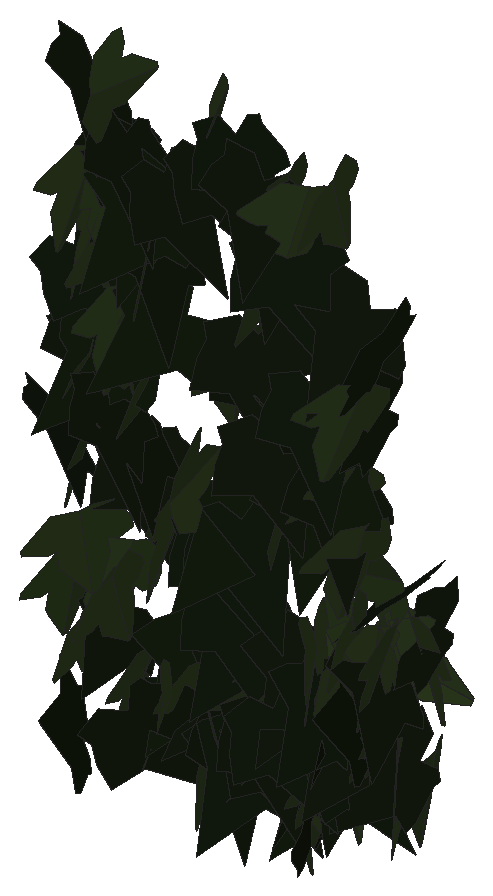
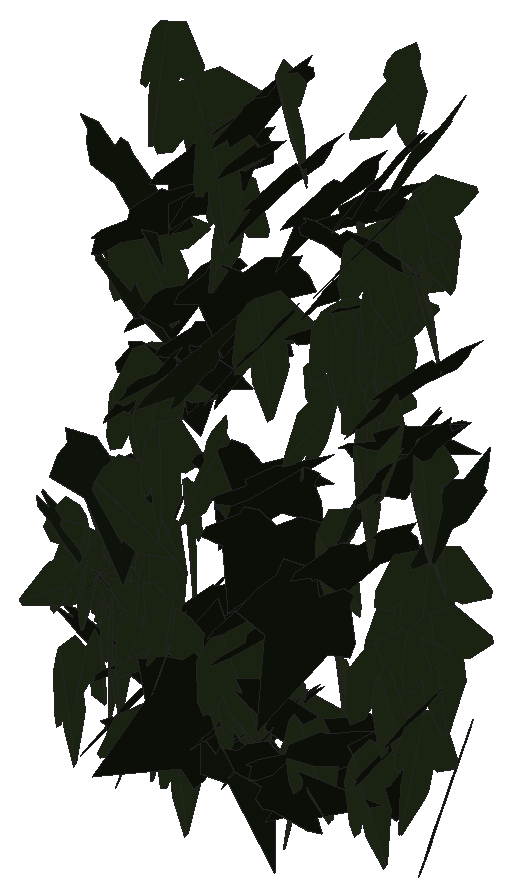
# SketchUp Ruby script. Lengths in inches.
U = 1.inch
M = Sketchup.active_model
def pt(a) = Geom::Point3d.new(a.map { |v| v * U })
def face(e, loops, mat)
  f = e.add_face(loops[0].map { |a| pt(a) })
  loops[1..].each { |l| e.add_face(l.map { |a| pt(a) }).erase! }
  f.material = f.back_material = mat if mat
  f
end
# faces: each face lists its corners as indices into pts; further lists are holes
def faces(e, pts, list, mat = nil) = list.each { |f| face(e, (f[0].is_a?(Array) ? f : [f]).map { |l| l.map { |i| pts[i] } }, mat) }
# xy, xz, yz: faces in a plane at the given z, y or x. An outline is a flat list of corners, or four numbers for a rectangle; further outlines are holes
def ring(l) = l.size == 4 ? [[l[0], l[1]], [l[2], l[1]], [l[2], l[3]], [l[0], l[3]]] : l.each_slice(2).to_a
def flat(e, list, mat, &to3) = list.each { |f| face(e, (f[0].is_a?(Array) ? f : [f]).map { |l| ring(l).map { |u, v| to3.(u, v) } }, mat) }
def xy(e, z, list, mat = nil) = flat(e, list, mat) { |x, y| [x, y, z] }
def xz(e, y, list, mat = nil) = flat(e, list, mat) { |x, z| [x, y, z] }
def yz(e, x, list, mat = nil) = flat(e, list, mat) { |y, z| [x, y, z] }
def lines(e, pts, list) = list.each { |a, b| e.add_line(pt(pts[a]), pt(pts[b])) }
# prism: a flat outline (further loops are holes) pulled along v
def prism(e, loops, v, mat = nil)
  f = face(e, loops, mat); d = Geom::Vector3d.new(v.map { |x| x * U })
  f.pushpull(f.normal.samedirection?(d) ? d.length : -d.length)
end
def box(e, o, s, mat = nil) = prism(e, [[o, [o[0] + s[0], o[1], o[2]], [o[0] + s[0], o[1] + s[1], o[2]], [o[0], o[1] + s[1], o[2]]]], [0, 0, s[2]], mat)
def at(x, y, z, deg = 0) = Geom::Transformation.translation(pt([x, y, z])) * Geom::Transformation.rotation(ORIGIN, Z_AXIS, deg.degrees)
def axes(o, x, y, z) = Geom::Transformation.new([*x, 0, *y, 0, *z, 0, *pt(o).to_a, 1])
def part(name) = M.definitions.add(name)
# library, detail: a bought-in or finely detailed component or shape, given as its bounding box
def library(name, o, s) = part(name).tap { |d| box(d.entities, o, s) }
def detail(e, o, s) = box(e.add_group.entities, o, s)
def put(e, d, t, mat = nil) = e.add_instance(d, t).tap { |i| i.material = mat if mat }
def group(e, t, mat = nil) = e.add_group.tap { |g| g.transformation = t; g.material = mat if mat }.entities
root = M.entities
M.materials.add("efeu1").color = [18, 25, 13]
M.materials.add("efeu2").color = [43, 57, 29]
c1 = part("ivyleaf_10")
p = [[0,0.5,-0.03],[-0.0625,2.02,-0.43],[-0.19,2.01,-0.46],[-0.54,1.05,-0.29],[-0.52,0.625,-0.18],[-0.83,0.76,-0.28],
  [-1.16,0.64,-0.33],[-1.15,0.33,-0.24],[-0.77,-0.39,0.02],[-0.3,-0.51,0.16],[0.04,-0.48,0.23],[-0.02,2.01,-0.4375],
  [-0.06,2.01,-0.43],[0.04,-0.49,0.23],[0.67,-0.49,0.14],[1.38,0.36,-0.2],[1.375,0.51,-0.24],[0.81,0.65,-0.19],
  [0.62,0.59,-0.15],[0.6,1.09,-0.28],[0.5,1.23,-0.31]]
faces(c1.entities,p,[[0,1,2,3,4,5,6,7,8,9,10],[11,12,0,13,14,15,16,17,18,19,20]],"efeu2")
c2 = part("ivyleaf_9")
p = [[1.54,2.16,1.25],[1.36,2.04,1.19],[-0.21,0.99,0.68],[-0.71,1.11,0.82],[-0.85,0.86,0.67],[-0.8,0.17,0.21],
  [-0.9,-0.01,0.1],[-0.67,-0.16,-0.02],[-0.08,-0.08,-0.05],[-0.03,-0.6,-0.4],[0.65,-0.88,-0.66],[0.83,-0.6,-0.49],
  [1.29,-0.42,-0.43],[1.8125,-0.07,-0.26],[1.21,0.44,0.15]]
faces(c2.entities,p,[[0,1,2,3,4,5,6,7,8,9,10,11,12,13,14]],"efeu1")
put(root,c1,axes([27.02,222.2,235.84],[0.27164,-0.32229,-0.26896],[-0.09984,0.26157,-0.41426],[0.40773,0.27877,0.07775]))
put(root,c2,axes([24.59,222.71,240.35],[-0.29862,-0.35269,0.19088],[-0.03799,-0.21204,-0.45121],[0.39923,-0.28399,0.09984]))
put(root,c1,axes([23.69,222.52,240.5625],[-0.01097,-0.47184,0.16507],[0.03742,-0.16543,-0.47036],[0.49848,0.00203,0.03894]))
put(root,c1,axes([24.21,222.51,239.03],[-0.03517,-0.47829,0.14144],[0.08713,-0.1455,-0.47036],[0.49109,-0.00844,0.09358]))
put(root,c2,axes([26.46,222.32,234.88],[0.08252,-0.39457,-0.29582],[-0.00101,0.29979,-0.40015],[0.49314,0.06664,0.04868]))
put(root,c1,axes([27.39,222.5,238.9375],[-0.15374,-0.44872,0.15817],[-0.03284,-0.15581,-0.47397],[0.47464,-0.15613,0.01844]))
put(root,c2,axes([26.36,222.43,238.18],[-0.08203,-0.40902,-0.27564],[0.09548,0.26097,-0.41566],[0.4839,-0.12083,0.03529]))
put(root,c2,axes([24.82,222.77,238.98],[-0.32782,-0.29622,0.23407],[-0.06945,-0.25739,-0.423],[0.37109,-0.30985,0.12761]))
put(root,c2,axes([25.96,222.71,241.03],[-0.03709,-0.47389,0.15508],[0.02325,-0.15698,-0.47415],[0.49808,-0.02796,0.03368]))
put(root,c1,axes([23.78,222.35,236.26],[-0.27606,-0.40929,-0.07917],[0.04487,0.06523,-0.49369],[0.41446,-0.27969,0.00071]))
put(root,c1,axes([24.96,222.26,234.52],[0.17602,-0.36599,-0.29167],[-0.13615,0.25809,-0.40602],[0.44775,0.22236,-0.0088]))
put(root,c1,axes([25.43,222.04,237.35],[0.02628,-0.01844,0.49897],[-0.24153,0.43684,0.02886],[-0.437,-0.24255,0.01406]))
put(root,c2,axes([27.27,222.76,234.82],[-0.08751,-0.04047,0.49062],[-0.0735,-0.49165,-0.05367],[0.48676,-0.08152,0.0801]))
put(root,c2,axes([23.18,222.71,237.16],[0.10075,-0.36999,0.32087],[0.15594,-0.28631,-0.3791],[0.46426,0.17646,0.0577]))
put(root,c2,axes([23.42,222.76,233.37],[-0.09246,-0.01791,0.49105],[-0.04589,-0.49717,-0.02677],[0.48923,-0.05002,0.0903]))
put(root,c2,axes([25.73,222.82,236.79],[-0.29562,-0.3588,0.18405],[-0.02742,-0.20979,-0.45303],[0.40231,-0.27794,0.10436]))
put(root,c2,axes([26.95,222.63,237.78],[-0.36102,-0.29576,-0.17942],[0.14103,0.11095,-0.46669],[0.31587,-0.38758,0.00331]))
put(root,c2,axes([23.9375,222.63,237.71],[0.15387,-0.47573,-0.00212],[-0.00062,0.00203,-0.5],[0.47574,0.15387,0.00003]))
put(root,c2,axes([26.78,222.54,233.38],[-0.01465,0.3683,0.33784],[-0.12204,-0.33039,0.35489],[0.48466,-0.07206,0.09958]))
put(root,c2,axes([26.75,222.65,238.7],[0.00917,-0.49319,-0.08172],[0.00753,0.08186,-0.4932],[0.49986,0.00781,0.00893]))
put(root,c1,axes([24.56,222.41,239.8125],[0.28014,-0.36912,-0.18781],[-0.06124,0.18733,-0.45952],[0.4096,0.28046,0.05975]))
put(root,c2,axes([27.91,222.3,239.73],[-0.23527,0.41139,0.15939],[-0.09462,0.12938,-0.47361],[-0.43092,-0.25301,0.01697]))
put(root,c2,axes([25.73,222.875,233.9],[-0.17539,-0.41991,0.20715],[-0.02601,-0.21213,-0.45202],[0.46751,-0.16933,0.05257]))
put(root,c1,axes([23.52,222.55,235.63],[-0.07759,-0.49393,-0.00373],[0.00149,0.00354,-0.49999],[0.49394,-0.0776,0.00092]))
put(root,c1,axes([27.36,222.6,237.19],[-0.09582,-0.48732,0.05775],[-0.01051,-0.05679,-0.49665],[0.49062,-0.0964,0.00064]))
put(root,c2,axes([26.71,222.93,234.78],[-0.12651,-0.36116,0.32181],[-0.01217,-0.33015,-0.3753],[0.48358,-0.1028,0.07474]))
put(root,c1,axes([24.2,222.43,239.84],[-0.18172,-0.43005,-0.17899],[0.05797,0.16976,-0.46671],[0.46219,-0.19037,-0.01184]))
put(root,c1,axes([26.44,222.81,233.54],[0.06044,-0.08595,-0.48883],[0.28794,-0.39504,0.10506],[-0.40428,-0.29421,0.00175]))
put(root,c2,axes([25.8,222.5625,236.86],[-0.20522,-0.25885,-0.37534],[0.24055,0.28819,-0.33027],[0.38732,-0.31614,0.00625]))
put(root,c2,axes([24.1,222.72,240.95],[0.13924,-0.48001,0.0141],[0.00413,-0.01348,-0.4998],[0.4802,0.1393,0.00021]))
put(root,c1,axes([24.16,222.19,241.82],[-0.00716,-0.11697,-0.48607],[0.08913,0.47804,-0.11635],[0.49194,-0.08831,0.014]))
put(root,c1,axes([24.12,222.45,235.57],[-0.02081,-0.45202,-0.21272],[0.03296,0.2112,-0.45201],[0.49848,-0.03284,0.02101]))
put(root,c1,axes([27.62,222.74,235.97],[0.21044,-0.43276,0.13578],[0.04232,-0.13029,-0.48087],[0.45158,0.21388,-0.01821]))
put(root,c2,axes([25.9375,222.68,239.12],[-0.12272,-0.42627,-0.23073],[0.06796,0.22053,-0.44356],[0.47992,-0.14023,0.00381]))
put(root,c1,axes([23.66,222.64,239.83],[0.31119,-0.39056,-0.02505],[-0.01242,0.02213,-0.49936],[0.39116,0.31141,0.00407]))
put(root,c2,axes([26.33,222.61,240.42],[0.0229,-0.42507,-0.26229],[0.01937,0.26312,-0.42473],[0.4991,0.00929,0.02851]))
put(root,c2,axes([24.4375,222.83,239.78],[0.07969,-0.48968,0.06217],[0.01451,-0.06062,-0.4961],[0.4934,0.08087,0.00455]))
put(root,c1,axes([26.52,222.71,240.99],[-0.26444,-0.4039,0.13012],[-0.03098,-0.13453,-0.48056],[0.42321,-0.26223,0.04612]))
put(root,c2,axes([26.95,222.83,237.68],[0.01658,-0.49941,-0.01778],[-0.00304,0.01769,-0.49968],[0.49972,0.01668,-0.00245]))
put(root,c1,axes([23.56,222.72,237.24],[0.25419,-0.42943,0.03129],[0.00758,-0.03187,-0.49893],[0.4305,0.25412,-0.00969]))
put(root,c2,axes([25.4375,222.9,233.99],[0.0901,-0.48493,0.08199],[0.00838,-0.08183,-0.49319],[0.49174,0.09025,-0.00662]))
put(root,c1,axes([27.04,222.56,241.38],[0.0352,-0.45479,-0.20476],[0.03648,0.20706,-0.45365],[0.49742,0.01699,0.04776]))
put(root,c2,axes([23.42,222.98,241.47],[0.07823,-0.44138,0.22151],[0.06292,-0.21354,-0.44771],[0.48982,0.09793,0.02213]))
put(root,c2,axes([25.98,222.78,234.43],[0.08024,-0.4752,-0.13322],[0.01057,0.13659,-0.48087],[0.49341,0.07435,0.03197]))
put(root,c2,axes([27.36,223.01,235.4375],[0.01548,-0.45973,0.19597],[0.03998,-0.1943,-0.45897],[0.49816,0.02988,0.03075]))
put(root,c2,axes([25.55,222.79,241.4],[0.11965,-0.47132,-0.11638],[-0.03302,0.11168,-0.48625],[0.48435,0.12404,-0.00441]))
put(root,c1,axes([24.27,222.81,239.03],[-0.07032,-0.48677,0.09007],[-0.01075,-0.08945,-0.49182],[0.49491,-0.0711,0.00211]))
put(root,c1,axes([24.61,222.92,236.46],[0.16594,-0.41447,0.22512],[0.0942,-0.20471,-0.44634],[0.46216,0.19054,0.01014]))
put(root,c2,axes([24.34,222.51,234.05],[-0.00426,-0.10556,-0.48871],[0.1696,0.45945,-0.10072],[0.47034,-0.16663,0.0319]))
put(root,c2,axes([26.4,223.09,235.16],[-0.19912,-0.42217,0.17922],[-0.03138,-0.18239,-0.46449],[0.45757,-0.19622,0.04614]))
put(root,c1,axes([26.16,222.55,239.93],[-0.00152,-0.40118,-0.29841],[0.00883,0.29835,-0.40114],[0.49992,-0.00648,0.00618]))
put(root,c1,axes([26.68,222.84,234.08],[0.12287,-0.4803,0.06492],[0.01082,-0.06424,-0.49574],[0.48455,0.12323,-0.00539]))
put(root,c2,axes([24.65,222.72,240.65],[0.17746,-0.40913,-0.2261],[-0.04041,0.22751,-0.4434],[0.4657,0.17565,0.04768]))
put(root,c1,axes([25.24,222.58,233.75],[0.23847,-0.3579,-0.25503],[0.01127,0.29504,-0.40351],[0.43932,0.1867,0.14879]))
put(root,c1,axes([27.02,222.67,237.65],[-0.20799,-0.43309,-0.13846],[0.04438,0.1322,-0.48016],[0.45252,-0.21203,-0.01655]))
put(root,c2,axes([23.79,223.11,238.13],[-0.38168,-0.28762,0.14695],[-0.03935,-0.18437,-0.4631],[0.32058,-0.36508,0.11811]))
put(root,c1,axes([25.87,223.01,234.43],[0.09197,-0.43323,0.23206],[0.04856,-0.22692,-0.44289],[0.48906,0.10401,0.00033]))
put(root,c2,axes([23.99,223.07,237.23],[0.1136,-0.44155,0.20526],[0.07031,-0.19369,-0.45557],[0.48182,0.13237,0.01809]))
put(root,c2,axes([27.52,222.85,238.73],[-0.43626,0.23355,-0.07163],[0.0525,-0.05355,-0.49434],[-0.23858,-0.43885,0.0222]))
put(root,c1,axes([23.95,222.88,240.24],[-0.25362,-0.41994,0.09658],[-0.03006,-0.09455,-0.49006],[0.42985,-0.25438,0.02271]))
put(root,c2,axes([27.02,223.17,239.62],[-0.20632,-0.42622,0.16053],[-0.03748,-0.15974,-0.47231],[0.4539,-0.20693,0.03397]))
put(root,c2,axes([26.99,223.21,234.49],[-0.23838,-0.38423,0.21341],[0.01579,-0.2501,-0.43266],[0.43923,-0.19954,0.13137]))
put(root,c1,axes([27.18,222.7,236.02],[0.1216,-0.42852,-0.22713],[0.03755,0.24178,-0.43604],[0.48353,0.08898,0.09098]))
put(root,c1,axes([25.55,222.86,238.77],[-0.02606,-0.49831,-0.03174],[0.00426,0.03156,-0.49898],[0.4993,-0.02628,0.00261]))
put(root,c2,axes([25.4375,223.22,235.23],[-0.18783,-0.40207,0.23035],[-0.03625,-0.23505,-0.43982],[0.46196,-0.18193,0.05915]))
put(root,c1,axes([23.43,222.82,237.86],[0.13554,-0.46575,-0.12125],[-0.00742,0.12393,-0.48434],[0.48122,0.13309,0.02668]))
put(root,c2,axes([27.85,222.97,234.49],[-0.49197,0.08493,0.02746],[-0.0303,-0.01423,-0.49888],[-0.08396,-0.49253,0.01914]))
put(root,c2,axes([25.36,222.95,235.66],[0.06604,-0.46846,-0.16182],[0.01995,0.16563,-0.47135],[0.49522,0.05579,0.04057]))
put(root,c2,axes([24.3,223.1,240.33],[-0.40209,-0.23417,-0.183],[0.20911,-0.00416,-0.45415],[0.21117,-0.44176,0.10128]))
put(root,c2,axes([25.92,223.15,240.43],[-0.04732,-0.49011,0.08689],[-0.01233,-0.0861,-0.49238],[0.4976,-0.04874,-0.00394]))
put(root,c1,axes([25.17,222.9375,241.61],[0.2641,-0.42453,0.00495],[0.00692,-0.00153,-0.49995],[0.42451,0.26414,0.00507]))
put(root,c1,axes([27.22,222.68,235.64],[-0.14191,-0.37108,-0.30358],[0.14343,0.26924,-0.39615],[0.45748,-0.19952,0.03004]))
put(root,c1,axes([24.125,222.86,238.49],[-0.00575,-0.48342,-0.12755],[0.02169,0.1272,-0.48306],[0.4995,-0.01109,0.01951]))
put(root,c1,axes([27.65,222.97,234.41],[-0.20131,0.43218,-0.15066],[-0.04278,-0.18164,-0.46387],[-0.45568,-0.17387,0.11011]))
put(root,c2,axes([25.31,222.96,236.48],[-0.14578,-0.32558,-0.35035],[0.17023,0.30696,-0.35608],[0.44696,-0.2231,0.02134]))
put(root,c2,axes([26.61,223.09,234.4],[-0.40732,0.12704,-0.26068],[0.2398,-0.10518,-0.42595],[-0.16306,-0.47202,0.02475]))
put(root,c1,axes([24.44,223.01,239.15],[-0.02324,-0.4994,0.00799],[0.00711,-0.00833,-0.49988],[0.49941,-0.02312,0.00748]))
put(root,c2,axes([26.11,222.95,238.28],[0.34962,-0.35348,-0.05303],[0.02517,0.09835,-0.48958],[0.35655,0.33967,0.08657]))
put(root,c2,axes([25.46,223.07,238.6],[0.18053,-0.46233,-0.06048],[-0.01331,0.05972,-0.49624],[0.46608,0.18078,0.00925]))
put(root,c1,axes([25.63,223.08,234.73],[0.01107,-0.49293,0.08305],[0.01057,-0.08282,-0.49298],[0.49977,0.01267,0.00859]))
put(root,c2,axes([26.8,222.87,234.3],[0.29453,-0.32576,-0.23903],[-0.06555,0.25335,-0.42605],[0.39869,0.2823,0.10653]))
put(root,c1,axes([23.75,223.12,235.49],[-0.18731,-0.4351,0.16002],[-0.00364,-0.1712,-0.46976],[0.46357,-0.17715,0.06097]))
put(root,c2,axes([26.09,223.16,234.45],[0.124,-0.17292,0.45247],[0.32623,-0.31543,-0.20995],[0.35805,0.34728,0.0346]))
put(root,c2,axes([23.74,222.93,240.7],[0.29046,-0.35723,-0.19498],[-0.03761,0.21496,-0.44986],[0.40524,0.276,0.09801]))
put(root,c2,axes([25.77,223,234.1],[0.16389,-0.42164,-0.21297],[-0.03438,0.21418,-0.45049],[0.47113,0.1623,0.04121]))
put(root,c1,axes([25.09,222.9,234.37],[-0.2654,0.42334,0.01845],[-0.00485,0.01873,-0.49963],[-0.42372,-0.26539,-0.00583]))
put(root,c2,axes([23.53,223.38,234.69],[-0.07232,-0.39441,0.29869],[-0.00942,-0.30071,-0.39936],[0.49465,-0.06339,0.03606]))
put(root,c2,axes([25.83,222.86,233.82],[-0.17082,0.46987,-0.00664],[0.00364,-0.00574,-0.49995],[-0.4699,-0.17086,-0.00146]))
put(root,c2,axes([23.32,223.27,238.16],[0.00944,-0.49977,0.01206],[0.00355,-0.01199,-0.49984],[0.4999,0.00952,0.00332]))
put(root,c1,axes([23.41,222.9,234.69],[0.01732,-0.43513,-0.24568],[0.0425,0.24622,-0.43309],[0.49789,-0.00589,0.04552]))
put(root,c2,axes([23.21,222.99,239.14],[0.21926,-0.38124,-0.23787],[0.03254,0.27745,-0.41468],[0.44818,0.16637,0.14647]))
put(root,c1,axes([27.36,223.01,234.77],[0.11827,-0.46785,-0.13089],[-0.02066,0.12975,-0.48243],[0.48537,0.11952,0.01136]))
put(root,c1,axes([23.63,223.17,235.19],[0.11637,-0.48045,0.07501],[0.01676,-0.07312,-0.49434],[0.48598,0.11756,-0.00091]))
put(root,c2,axes([26.53,223.36,234.16],[-0.0283,-0.4772,0.14655],[0.0355,-0.14834,-0.47617],[0.49793,-0.01654,0.04228]))
put(root,c1,axes([24.72,223.17,234.37],[0.06374,-0.49134,0.06722],[-0.00042,-0.06782,-0.49538],[0.49592,0.0631,-0.00906]))
put(root,c2,axes([24.95,223.03,240.88],[0.22383,-0.39056,-0.21764],[-0.02579,0.23171,-0.44232],[0.44636,0.20923,0.08358]))
put(root,c2,axes([27.5625,222.8,236.36],[-0.01106,0.48349,0.12695],[-0.12732,0.12007,-0.46837],[-0.48339,-0.04269,0.12046]))
put(root,c1,axes([26.17,222.76,236.99],[0.04091,-0.17753,-0.46563],[0.0023,0.46726,-0.17795],[0.49832,0.01242,0.03905]))
put(root,c1,axes([24.05,223.06,237.77],[0.16571,-0.4554,-0.1231],[-0.01968,0.12368,-0.48406],[0.47133,0.16528,0.02307]))
put(root,c2,axes([24.01,223.2,236.82],[0.00186,-0.46111,-0.19333],[0.06598,0.19187,-0.45698],[0.49562,-0.02381,0.06156]))
put(root,c1,axes([26.8,223.09,235.48],[0.11925,-0.4748,-0.10169],[0.04532,0.11514,-0.48445],[0.48345,0.10632,0.0705]))
put(root,c2,axes([25.38,223.31,234.64],[-0.49232,-0.08536,0.01824],[-0.01971,0.00697,-0.49956],[0.08503,-0.49261,-0.01023]))
put(root,c1,axes([23.49,223.28,238.4375],[-0.21596,0.28894,-0.34623],[0.20453,-0.27937,-0.36072],[-0.4019,-0.29743,0.00247]))
put(root,c1,axes([25.92,223.125,240.82],[0.02119,-0.49246,-0.08389],[-0.01575,0.08327,-0.49277],[0.4993,0.02353,-0.01198]))
put(root,c1,axes([26.625,223.14,237.05],[0.05442,-0.48301,-0.11722],[0.01439,0.1194,-0.48532],[0.49682,0.04945,0.0269]))
put(root,c1,axes([25.6,223.32,235.05],[-0.11345,-0.46787,0.13499],[-0.02614,-0.13255,-0.4814],[0.48626,-0.11629,0.00562]))
put(root,c2,axes([26.62,223.45,233.98],[-0.40359,-0.29144,0.04669],[-0.04023,-0.02404,-0.4978],[0.2924,-0.40557,-0.00405]))
put(root,c1,axes([23.88,223.29,234.2],[0.11241,-0.48496,0.04669],[0.00466,-0.04685,-0.49778],[0.48718,0.11234,-0.00602]))
put(root,c1,axes([27.26,223.11,234.78],[0.17631,-0.43112,-0.18179],[0.01169,0.19827,-0.45886],[0.46774,0.15755,0.08]))
put(root,c1,axes([26.71,223.13,234.29],[0.13111,-0.42512,-0.22823],[-0.02931,0.22905,-0.44348],[0.48161,0.12967,0.03513]))
put(root,c1,axes([26.67,223.24,234.11],[-0.14195,0.47205,-0.08378],[0.04089,-0.07514,-0.49263],[-0.47768,-0.14671,-0.01728]))
put(root,c1,axes([26.29,223.3125,233.84],[0.06691,-0.49071,-0.06876],[-0.00354,0.06891,-0.49522],[0.49549,0.06676,0.00575]))
put(root,c2,axes([24.54,223.67,234.42],[-0.2888,-0.39112,0.1167],[-0.0001,-0.14289,-0.47915],[0.40816,-0.27678,0.08246]))
put(root,c2,axes([27.85,223.38,235.94],[-0.4392,0.23226,-0.05621],[0.03533,-0.05319,-0.49591],[-0.23634,-0.43957,0.03031]))
put(root,c1,axes([27.32,223.25,235.71],[-0.11666,0.48453,0.04021],[-0.00834,0.03935,-0.49838],[-0.48613,-0.11695,-0.0011]))
put(root,c1,axes([26.45,223.31,235.18],[0.38464,0.09175,0.306],[0.28164,0.12864,-0.39259],[-0.15077,0.47438,0.04728]))
put(root,c1,axes([27.68,223.41,234.17],[0.14566,-0.47778,-0.02268],[0.03667,0.03479,-0.49744],[0.47691,0.14325,0.04518]))
put(root,c2,axes([25.09,223.37,233.71],[-0.20321,0.12512,0.43938],[-0.42288,0.13045,-0.23272],[-0.17287,-0.46619,0.0528]))
put(root,c1,axes([27.61,223.36,235.79],[-0.40038,0.28731,-0.08452],[0.05594,-0.06689,-0.49234],[-0.29422,-0.4037,0.02142]))
put(root,c1,axes([27.16,223.27,236.36],[0.16427,0.07051,-0.46695],[-0.43348,0.21867,-0.11948],[0.18737,0.44408,0.13297]))
put(root,c1,axes([26.45,223.53,234.16],[0.27454,0.36184,-0.20905],[-0.1143,-0.17558,-0.45399],[-0.40195,0.29706,-0.01369]))
put(root,c1,axes([27.23,223.25,235.44],[0.15501,0.12329,0.4591],[0.34082,0.3078,-0.19774],[-0.33138,0.37424,0.01138]))
put(root,c1,axes([26.28,223.48,235.45],[-0.09758,0.4903,-0.00932],[-0.03203,-0.01585,-0.49872],[-0.48934,-0.09673,0.0345]))
put(root,c2,axes([26.36,223.44,234.85],[0.2926,-0.16253,-0.37145],[-0.3173,0.19337,-0.33455],[0.2524,0.4315,0.01002]))
put(root,c2,axes([24.3,223.55,236.24],[0.42651,0.20166,-0.16559],[-0.1914,0.02612,-0.46117],[-0.17735,0.45678,0.09948]))
put(root,c2,axes([25.96,223.41,234.29],[0.18707,0.29,0.36181],[0.20813,0.29612,-0.34496],[-0.41435,0.27967,-0.00993]))
